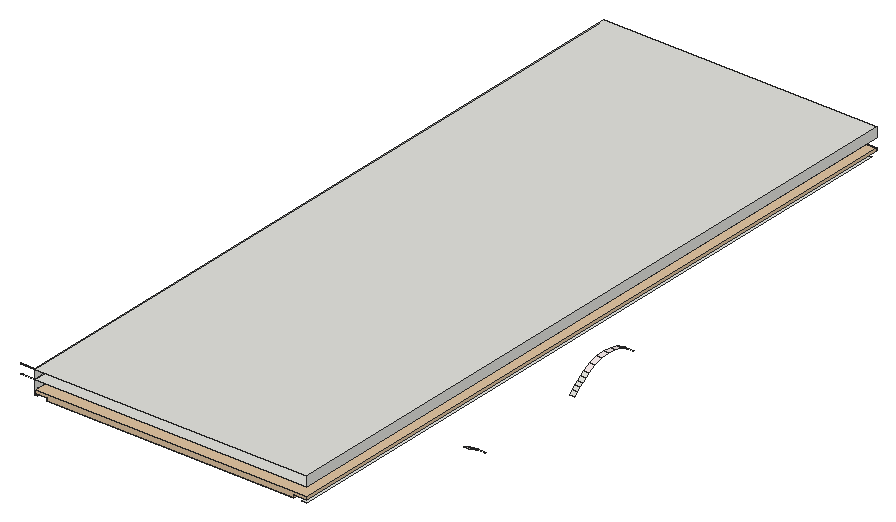
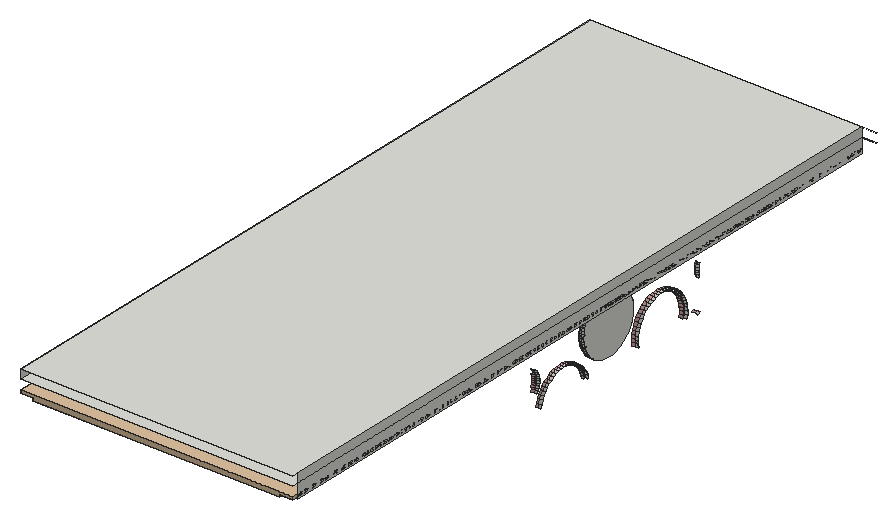
# SketchUp Ruby script. Lengths in inches.
U = 1.inch
M = Sketchup.active_model
def pt(a) = Geom::Point3d.new(a.map { |v| v * U })
def face(e, loops, mat)
  f = e.add_face(loops[0].map { |a| pt(a) })
  loops[1..].each { |l| e.add_face(l.map { |a| pt(a) }).erase! }
  f.material = f.back_material = mat if mat
  f
end
# faces: each face lists its corners as indices into pts; further lists are holes
def faces(e, pts, list, mat = nil) = list.each { |f| face(e, (f[0].is_a?(Array) ? f : [f]).map { |l| l.map { |i| pts[i] } }, mat) }
# xy, xz, yz: faces in a plane at the given z, y or x. An outline is a flat list of corners, or four numbers for a rectangle; further outlines are holes
def ring(l) = l.size == 4 ? [[l[0], l[1]], [l[2], l[1]], [l[2], l[3]], [l[0], l[3]]] : l.each_slice(2).to_a
def flat(e, list, mat, &to3) = list.each { |f| face(e, (f[0].is_a?(Array) ? f : [f]).map { |l| ring(l).map { |u, v| to3.(u, v) } }, mat) }
def xy(e, z, list, mat = nil) = flat(e, list, mat) { |x, y| [x, y, z] }
def xz(e, y, list, mat = nil) = flat(e, list, mat) { |x, z| [x, y, z] }
def yz(e, x, list, mat = nil) = flat(e, list, mat) { |y, z| [x, y, z] }
def lines(e, pts, list) = list.each { |a, b| e.add_line(pt(pts[a]), pt(pts[b])) }
# prism: a flat outline (further loops are holes) pulled along v
def prism(e, loops, v, mat = nil)
  f = face(e, loops, mat); d = Geom::Vector3d.new(v.map { |x| x * U })
  f.pushpull(f.normal.samedirection?(d) ? d.length : -d.length)
end
def box(e, o, s, mat = nil) = prism(e, [[o, [o[0] + s[0], o[1], o[2]], [o[0] + s[0], o[1] + s[1], o[2]], [o[0], o[1] + s[1], o[2]]]], [0, 0, s[2]], mat)
def at(x, y, z, deg = 0) = Geom::Transformation.translation(pt([x, y, z])) * Geom::Transformation.rotation(ORIGIN, Z_AXIS, deg.degrees)
def axes(o, x, y, z) = Geom::Transformation.new([*x, 0, *y, 0, *z, 0, *pt(o).to_a, 1])
def part(name) = M.definitions.add(name)
# library, detail: a bought-in or finely detailed component or shape, given as its bounding box
def library(name, o, s) = part(name).tap { |d| box(d.entities, o, s) }
def detail(e, o, s) = box(e.add_group.entities, o, s)
def put(e, d, t, mat = nil) = e.add_instance(d, t).tap { |i| i.material = mat if mat }
def group(e, t, mat = nil) = e.add_group.tap { |g| g.transformation = t; g.material = mat if mat }.entities
root = M.entities
M.materials.add("Generic").color = [224, 169, 169]
M.materials.add("Generic\#2").color = [246, 234, 234]
M.materials.add("Generic\#3").color = [224, 196, 161]
M.materials.add("[Mirror 01]").color = [185, 185, 185]
xy(root,120,[[180.9375,0,184.0625,453.375],[9,0.4375,10.6875,0.4375,10.6875,106.01,11.4375,106.01,11.4375,107.97,10.6875,107.97,10.6875,125.48,11.4375,125.48,11.4375,127.43,10.6875,127.43,10.6875,185.75,12.375,185.75,12.375,188.375,10.6875,188.375,10.6875,218.875,12.375,218.875,12.375,221.5,10.6875,221.5,10.6875,295.22,12.1875,295.22,12.1875,297.72,10.6875,297.72,10.6875,330.66,12.1875,330.66,12.1875,333.16,10.6875,333.16,10.6875,453.375,9,453.375]])
xy(root,129.25,[[0,0,0,0.4375,9,0.4375,9,457.3,184.0625,457.3,184.0625,0]])
xy(root,135.25,[[0,0,184.0625,0,184.0625,457.3,9,457.3,9,0.4375,0,0.4375]])
yz(root,9,[[203.625,92.14,205.19,92.2,206.74,92.38,208.27,92.69,209.77,93.12,211.23,93.67,212.64,94.33,214,95.1,215.29,95.97,216.51,96.95,217.65,98.02,218.7,99.17,219.66,100.41,220.51,101.71,221.26,103.08,221.89,104.51,222.42,105.98,222.82,107.49,223.1,109.02,223.26,110.58,223.3,112.14,223.21,113.7,223,115.24,222.66,116.77,222.21,118.26,221.64,119.71,221.5,120,185.75,120,185.61,119.71,185.04,118.26,184.59,116.77,184.25,115.24,184.04,113.7,183.95,112.14,183.99,110.58,184.15,109.02,184.43,107.49,184.84,105.98,185.36,104.51,185.99,103.08,186.74,101.71,187.6,100.41,188.55,99.17,189.6,98.02,190.74,96.95,191.96,95.97,193.25,95.1,194.61,94.33,196.02,93.67,197.48,93.12,198.99,92.69,200.52,92.38,202.07,92.2],[0.4375,120,453.375,129.25],[0.4375,129.25,453.375,135.25]])
yz(root,10.6875,[[203.625,94.5,205,94.55,206.36,94.72,207.71,94.99,209.03,95.37,210.32,95.85,211.5625,96.43,212.76,97.1,213.89,97.875,214.97,98.73,215.97,99.67,216.89,100.6875,217.73,101.78,218.48,102.93,219.14,104.13,219.7,105.39,220.16,106.68,220.51,108.01,220.76,109.36,220.9,110.72,220.93,112.1,220.86,113.47,220.67,114.83,220.375,116.17,219.98,117.49,219.48,118.77,218.875,120,188.375,120,187.77,118.77,187.27,117.49,186.875,116.17,186.58,114.83,186.4,113.47,186.32,112.1,186.35,110.72,186.49,109.36,186.74,108.01,187.09,106.68,187.55,105.39,188.11,104.13,188.77,102.93,189.52,101.78,190.36,100.6875,191.28,99.67,192.29,98.73,193.36,97.875,194.5,97.1,195.69,96.43,196.93,95.85,198.22,95.37,199.54,94.99,200.89,94.72,202.25,94.55]],"[Mirror 01]")
yz(root,12.375,[[203.625,92.14,205.19,92.2,206.74,92.38,208.27,92.69,209.77,93.12,211.23,93.67,212.64,94.33,214,95.1,215.29,95.97,216.51,96.95,217.65,98.02,218.7,99.17,219.66,100.41,220.51,101.71,221.26,103.08,221.89,104.51,222.42,105.98,222.82,107.49,223.1,109.02,223.26,110.58,223.3,112.14,223.21,113.7,223,115.24,222.66,116.77,222.21,118.26,221.64,119.71,221.5,120,218.875,120,219.48,118.77,219.98,117.49,220.375,116.17,220.67,114.83,220.86,113.47,220.93,112.1,220.9,110.72,220.76,109.36,220.51,108.01,220.16,106.68,219.7,105.39,219.14,104.13,218.48,102.93,217.73,101.78,216.89,100.6875,215.97,99.67,214.97,98.73,213.89,97.875,212.76,97.1,211.5625,96.43,210.32,95.85,209.03,95.37,207.71,94.99,206.36,94.72,205,94.55,203.625,94.5,202.25,94.55,200.89,94.72,199.54,94.99,198.22,95.37,196.93,95.85,195.69,96.43,194.5,97.1,193.36,97.875,192.29,98.73,191.28,99.67,190.36,100.6875,189.52,101.78,188.77,102.93,188.11,104.13,187.55,105.39,187.09,106.68,186.74,108.01,186.49,109.36,186.35,110.72,186.32,112.1,186.4,113.47,186.58,114.83,186.875,116.17,187.27,117.49,187.77,118.77,188.375,120,185.75,120,185.61,119.71,185.04,118.26,184.59,116.77,184.25,115.24,184.04,113.7,183.95,112.14,183.99,110.58,184.15,109.02,184.43,107.49,184.84,105.98,185.36,104.51,185.99,103.08,186.74,101.71,187.6,100.41,188.55,99.17,189.6,98.02,190.74,96.95,191.96,95.97,193.25,95.1,194.61,94.33,196.02,93.67,197.48,93.12,198.99,92.69,200.52,92.38,202.07,92.2]],"Generic")
yz(root,184.0625,[[0,129.25,457.3,135.25]])
p = [[10.6875,131.75,85.21],[10.6875,130.28,85.99],[9,130.28,85.99],[9,131.75,85.21],[12.9375,130.28,85.99],[12.9375,131.75,85.21],
  [184.0625,143.35,85.58],[184.0625,140.15,87.99],[180.9375,140.15,87.99],[180.9375,143.35,85.58],[10.6875,256.25,88.14],[10.6875,256.74,86.13],
  [12.1875,256.74,86.13],[12.1875,256.25,88.14],[184.0625,217.14,88.18],[184.0625,214.93,86.28],[180.9375,214.93,86.28],[180.9375,217.14,88.18],
  [10.6875,257.93,86.34],[10.6875,257.41,88.49],[9,257.41,88.49],[9,257.93,86.34],[12.1875,257.41,88.49],[12.1875,257.93,86.34],
  [10.6875,140.51,88.69],[10.6875,140.86,86.45],[9,140.86,86.45],[9,140.51,88.69],[13,140.86,86.45],[13,140.51,88.69],
  [10.6875,142.23,86.75],[10.6875,141.9,88.83],[13,141.9,88.83],[13,142.23,86.75],[10.6875,179.76,86.9],[10.6875,180.06,89.14],
  [9,180.06,89.14],[9,179.76,86.9],[13,180.06,89.14],[13,179.76,86.9],[10.6875,221.22,86.86],[10.6875,221.78,88.85],
  [12.1875,221.78,88.85],[12.1875,221.22,86.86],[10.6875,220.64,89.25],[10.6875,220.03,87.125],[9,220.03,87.125],[9,220.64,89.25],
  [12.1875,220.03,87.125],[12.1875,220.64,89.25],[10.6875,178.66,89.25],[10.6875,178.39,87.16],[13,178.39,87.16],[13,178.66,89.25],
  [184.0625,136.83,90.22],[180.9375,136.83,90.22],[10.6875,255.54,90.08],[12.1875,255.54,90.08],[184.0625,219.41,90.01],[180.9375,219.41,90.01],
  [10.6875,256.66,90.5625],[9,256.66,90.5625],[12.1875,256.66,90.5625],[10.6875,140.42,90.96],[9,140.42,90.96],[13,140.42,90.96],
  [10.6875,141.82,90.93],[13,141.82,90.93],[10.6875,222.57,90.76],[12.1875,222.57,90.76],[10.6875,180.1,91.41],[9,180.1,91.41],
  [13,180.1,91.41],[10.6875,178.7,91.35],[13,178.7,91.35],[10.6875,221.48,91.29],[9,221.48,91.29],[12.1875,221.48,91.29],
  [184.0625,221.73,91.77],[180.9375,221.73,91.77],[10.6875,254.61,91.93],[12.1875,254.61,91.93],[184.0625,133.39,92.26],[180.9375,133.39,92.26],
  [10.6875,255.67,92.54],[9,255.67,92.54],[12.1875,255.67,92.54],[10.6875,223.58,92.57],[12.1875,223.58,92.57],[10.6875,141.98,93.03],
  [13,141.98,93.03],[10.6875,140.59,93.22],[9,140.59,93.22],[13,140.59,93.22],[10.6875,222.55,93.22],[9,222.55,93.22],
  [12.1875,222.55,93.22],[10.6875,178.49,93.45],[13,178.49,93.45],[10.6875,179.88,93.66],[9,179.88,93.66],[13,179.88,93.66],
  [184.0625,224.11,93.46],[180.9375,224.11,93.46],[10.6875,253.48,93.66],[12.1875,253.48,93.66],[184.0625,262.21,91.98],[184.0625,257.84,95.3125],
  [180.9375,257.84,95.3125],[180.9375,262.21,91.98],[10.6875,202.07,92.2],[10.6875,203.625,92.14],[9,203.625,92.14],[9,202.07,92.2],
  [12.375,203.625,92.14],[12.375,202.07,92.2],[10.6875,205.19,92.2],[9,205.19,92.2],[12.375,205.19,92.2],[10.6875,200.52,92.38],
  [9,200.52,92.38],[12.375,200.52,92.38],[10.6875,206.74,92.38],[9,206.74,92.38],[12.375,206.74,92.38],[184.0625,129.85,94.12],
  [180.9375,129.85,94.12],[10.6875,198.99,92.69],[9,198.99,92.69],[12.375,198.99,92.69],[10.6875,208.27,92.69],[9,208.27,92.69],
  [12.375,208.27,92.69],[10.6875,254.46,94.39],[9,254.46,94.39],[12.1875,254.46,94.39],[10.6875,224.78,94.26],[12.1875,224.78,94.26],
  [10.6875,197.48,93.12],[9,197.48,93.12],[12.375,197.48,93.12],[10.6875,209.77,93.12],[9,209.77,93.12],[12.375,209.77,93.12],
  [10.6875,142.37,95.1],[13,142.37,95.1],[10.6875,196.02,93.67],[9,196.02,93.67],[12.375,196.02,93.67],[10.6875,211.23,93.67],
  [9,211.23,93.67],[12.375,211.23,93.67],[10.6875,141.01,95.44],[9,141.01,95.44],[13,141.01,95.44],[10.6875,223.83,95.02],
  [9,223.83,95.02],[12.1875,223.83,95.02],[10.6875,178.05,95.51],[13,178.05,95.51],[184.0625,226.54,95.08],[180.9375,226.54,95.08],
  [10.6875,179.4,95.88],[9,179.4,95.88],[13,179.4,95.88],[10.6875,194.61,94.33],[9,194.61,94.33],[12.375,194.61,94.33],
  [10.6875,212.64,94.33],[9,212.64,94.33],[12.375,212.64,94.33],[10.6875,252.16,95.26],[12.1875,252.16,95.26],[10.6875,193.25,95.1],
  [9,193.25,95.1],[12.375,193.25,95.1],[10.6875,214,95.1],[9,214,95.1],[12.375,214,95.1],[10.6875,226.17,95.79],
  [12.1875,226.17,95.79],[10.6875,253.05,96.08],[9,253.05,96.08],[12.1875,253.05,96.08],[10.6875,203.625,94.5],[10.6875,202.25,94.55],
  [12.375,202.25,94.55],[12.375,203.625,94.5],[10.6875,205,94.55],[12.375,205,94.55],[10.6875,200.89,94.72],[12.375,200.89,94.72],
  [10.6875,206.36,94.72],[12.375,206.36,94.72],[10.6875,199.54,94.99],[12.375,199.54,94.99],[10.6875,207.71,94.99],[12.375,207.71,94.99],
  [10.6875,198.22,95.37],[12.375,198.22,95.37],[10.6875,209.03,95.37],[12.375,209.03,95.37],[10.6875,225.3125,96.66],[9,225.3125,96.66],
  [12.1875,225.3125,96.66],[10.6875,143,97.11],[13,143,97.11],[10.6875,191.96,95.97],[9,191.96,95.97],[12.375,191.96,95.97],
  [10.6875,215.29,95.97],[9,215.29,95.97],[12.375,215.29,95.97],[184.0625,231.42,97.61],[180.9375,231.42,97.61],[10.6875,250.66,96.6875],
  [12.1875,250.66,96.6875],[184.0625,252.92,97.77],[180.9375,252.92,97.77],[10.6875,141.6875,97.61],[9,141.6875,97.61],[13,141.6875,97.61],
  [10.6875,196.93,95.85],[12.375,196.93,95.85],[10.6875,210.32,95.85],[12.375,210.32,95.85],[10.6875,177.38,97.5],[13,177.38,97.5],
  [10.6875,195.69,96.43],[12.375,195.69,96.43],[10.6875,211.5625,96.43],[12.375,211.5625,96.43],[10.6875,227.72,97.16],[12.1875,227.72,97.16],
  [10.6875,178.68,98.03],[9,178.68,98.03],[13,178.68,98.03],[10.6875,190.74,96.95],[9,190.74,96.95],[12.375,190.74,96.95],
  [10.6875,216.51,96.95],[9,216.51,96.95],[12.375,216.51,96.95],[10.6875,251.45,97.61],[9,251.45,97.61],[12.1875,251.45,97.61],
  [10.6875,260.36,97.44],[10.6875,261.03,96.23],[9,261.03,96.23],[9,260.36,97.44],[12.9375,261.03,96.23],[12.9375,260.36,97.44],
  [10.6875,194.5,97.1],[12.375,194.5,97.1],[10.6875,212.76,97.1],[12.375,212.76,97.1],[10.6875,226.97,98.12],[9,226.97,98.12],
  [12.1875,226.97,98.12],[10.6875,249.01,97.9375],[12.1875,249.01,97.9375],[10.6875,189.6,98.02],[9,189.6,98.02],[12.375,189.6,98.02],
  [10.6875,217.65,98.02],[9,217.65,98.02],[12.375,217.65,98.02],[10.6875,143.85,99.04],[13,143.85,99.04],[10.6875,193.36,97.875],
  [12.375,193.36,97.875],[10.6875,213.89,97.875],[12.375,213.89,97.875],[10.6875,229.42,98.34],[12.1875,229.42,98.34],[10.6875,259.83,98.73],
  [9,259.83,98.73],[12.9375,259.83,98.73],[10.6875,176.48,99.41],[13,176.48,99.41],[10.6875,142.61,99.68],[9,142.61,99.68],
  [13,142.61,99.68],[184.0625,236.6875,99.18],[180.9375,236.6875,99.18],[10.6875,249.69,98.95],[9,249.69,98.95],[12.1875,249.69,98.95],
  [184.0625,247.63,99.26],[180.9375,247.63,99.26],[10.6875,192.29,98.73],[12.375,192.29,98.73],[10.6875,214.97,98.73],[12.375,214.97,98.73],
  [10.6875,247.23,98.99],[12.1875,247.23,98.99],[10.6875,177.71,100.08],[9,177.71,100.08],[13,177.71,100.08],[10.6875,188.55,99.17],
  [9,188.55,99.17],[12.375,188.55,99.17],[10.6875,218.7,99.17],[9,218.7,99.17],[12.375,218.7,99.17],[10.6875,228.78,99.38],
  [9,228.78,99.38],[12.1875,228.78,99.38],[10.6875,231.24,99.32],[12.1875,231.24,99.32],[10.6875,191.28,99.67],[12.375,191.28,99.67],
  [10.6875,215.97,99.67],[12.375,215.97,99.67],[10.6875,259.45,100.07],[9,259.45,100.07],[12.9375,259.45,100.07],[10.6875,247.79,100.07],
  [9,247.79,100.07],[12.1875,247.79,100.07],[10.6875,144.92,100.86],[13,144.92,100.86],[10.6875,245.34,99.84],[12.1875,245.34,99.84],
  [10.6875,187.6,100.41],[9,187.6,100.41],[12.375,187.6,100.41],[10.6875,219.66,100.41],[9,219.66,100.41],[12.375,219.66,100.41],
  [184.0625,242.16,99.73],[180.9375,242.16,99.73],[10.6875,261.07,99.16],[10.6875,260.73,100.35],[12.9375,260.73,100.35],[12.9375,261.07,99.16],
  [10.6875,233.16,100.09],[12.1875,233.16,100.09],[10.6875,175.375,101.2],[13,175.375,101.2],[10.6875,230.73,100.42],[9,230.73,100.42],
  [12.1875,230.73,100.42],[10.6875,143.75,101.63],[9,143.75,101.63],[13,143.75,101.63],[10.6875,190.36,100.6875],[12.375,190.36,100.6875],
  [10.6875,216.89,100.6875],[12.375,216.89,100.6875],[10.6875,243.37,100.46],[12.1875,243.37,100.46],[10.6875,176.52,102.01],[9,176.52,102.01],
  [13,176.52,102.01],[10.6875,235.16,100.63],[12.1875,235.16,100.63],[10.6875,245.78,100.97],[9,245.78,100.97],[12.1875,245.78,100.97],
  [10.6875,259.23,101.44],[9,259.23,101.44],[12.9375,259.23,101.44],[10.6875,186.74,101.71],[9,186.74,101.71],[12.375,186.74,101.71],
  [10.6875,220.51,101.71],[9,220.51,101.71],[12.375,220.51,101.71],[10.6875,232.78,101.24],[9,232.78,101.24],[12.1875,232.78,101.24],
  [10.6875,260.53,101.58],[12.9375,260.53,101.58],[10.6875,241.34,100.86],[12.1875,241.34,100.86],[10.6875,237.21,100.94],[12.1875,237.21,100.94],
  [10.6875,189.52,101.78],[12.375,189.52,101.78],[10.6875,217.73,101.78],[12.375,217.73,101.78],[10.6875,146.1875,102.54],[13,146.1875,102.54],
  [10.6875,239.28,101.02],[12.1875,239.28,101.02],[10.6875,243.67,101.64],[9,243.67,101.64],[12.1875,243.67,101.64],[10.6875,174.07,102.85],
  [13,174.07,102.85],[10.6875,234.91,101.82],[9,234.91,101.82],[12.1875,234.91,101.82],[10.6875,259.17,102.83],[9,259.17,102.83],
  [12.9375,259.17,102.83],[10.6875,145.12,103.44],[9,145.12,103.44],[13,145.12,103.44],[10.6875,241.5,102.06],[9,241.5,102.06],
  [12.1875,241.5,102.06],[10.6875,260.47,102.82],[12.9375,260.47,102.82],[10.6875,185.99,103.08],[9,185.99,103.08],[12.375,185.99,103.08],
  [10.6875,221.26,103.08],[9,221.26,103.08],[12.375,221.26,103.08],[10.6875,188.77,102.93],[12.375,188.77,102.93],[10.6875,218.48,102.93],
  [12.375,218.48,102.93],[10.6875,237.09,102.15],[9,237.09,102.15],[12.1875,237.09,102.15],[10.6875,175.12,103.78],[9,175.12,103.78],
  [13,175.12,103.78],[10.6875,239.3,102.23],[9,239.3,102.23],[12.1875,239.3,102.23],[10.6875,147.64,104.07],[13,147.64,104.07],
  [10.6875,259.26,104.22],[9,259.26,104.22],[12.9375,259.26,104.22],[10.6875,260.56,104.06],[12.9375,260.56,104.06],[10.6875,172.58,104.35],
  [13,172.58,104.35],[10.6875,188.11,104.13],[12.375,188.11,104.13],[10.6875,219.14,104.13],[12.375,219.14,104.13],[10.6875,185.36,104.51],
  [9,185.36,104.51],[12.375,185.36,104.51],[10.6875,221.89,104.51],[9,221.89,104.51],[12.375,221.89,104.51],[10.6875,146.68,105.09],
  [9,146.68,105.09],[13,146.68,105.09],[10.6875,173.52,105.39],[9,173.52,105.39],[13,173.52,105.39],[10.6875,149.25,105.42],
  [13,149.25,105.42],[10.6875,187.55,105.39],[12.375,187.55,105.39],[10.6875,219.7,105.39],[12.375,219.7,105.39],[10.6875,260.78,105.28],
  [12.9375,260.78,105.28],[10.6875,259.51,105.59],[9,259.51,105.59],[12.9375,259.51,105.59],[10.6875,170.9375,105.66],[13,170.9375,105.66],
  [10.6875,184.84,105.98],[9,184.84,105.98],[12.375,184.84,105.98],[10.6875,222.42,105.98],[9,222.42,105.98],[12.375,222.42,105.98],
  [10.6875,148.42,106.54],[9,148.42,106.54],[13,148.42,106.54],[10.6875,261.14,106.47],[12.9375,261.14,106.47],[10.6875,151.01,106.58],
  [13,151.01,106.58],[10.6875,171.75,106.81],[9,171.75,106.81],[13,171.75,106.81],[10.6875,187.09,106.68],[12.375,187.09,106.68],
  [10.6875,220.16,106.68],[12.375,220.16,106.68],[10.6875,259.92,106.92],[9,259.92,106.92],[12.9375,259.92,106.92],[10.6875,169.15,106.78],
  [13,169.15,106.78],[10.6875,184.43,107.49],[9,184.43,107.49],[12.375,184.43,107.49],[10.6875,222.82,107.49],[9,222.82,107.49],
  [12.375,222.82,107.49],[10.6875,130.9,106.11],[10.6875,131.2,107.5],[9,131.2,107.5],[9,130.9,106.11],[11.4375,131.2,107.5],
  [11.4375,130.9,106.11],[10.6875,150.31,107.79],[9,150.31,107.79],[13,150.31,107.79],[10.6875,152.89,107.53],[13,152.89,107.53],
  [10.6875,186.74,108.01],[12.375,186.74,108.01],[10.6875,220.51,108.01],[12.375,220.51,108.01],[10.6875,167.25,107.69],[13,167.25,107.69],
  [10.6875,169.83,108.01],[9,169.83,108.01],[13,169.83,108.01],[10.6875,260.47,108.19],[9,260.47,108.19],[12.9375,260.47,108.19],
  [10.6875,131.375,108.91],[9,131.375,108.91],[11.4375,131.375,108.91],[10.6875,154.87,108.26],[13,154.87,108.26],[10.6875,184.15,109.02],
  [9,184.15,109.02],[12.375,184.15,109.02],[10.6875,223.1,109.02],[9,223.1,109.02],[12.375,223.1,109.02],[10.6875,165.26,108.375],
  [13,165.26,108.375],[10.6875,152.33,108.8125],[9,152.33,108.8125],[13,152.33,108.8125],[10.6875,167.78,108.99],[9,167.78,108.99],
  [13,167.78,108.99],[10.6875,186.49,109.36],[12.375,186.49,109.36],[10.6875,220.76,109.36],[12.375,220.76,109.36],[10.6875,261.17,109.4],
  [9,261.17,109.4],[12.9375,261.17,109.4],[10.6875,156.91,108.76],[13,156.91,108.76],[10.6875,163.2,108.83],[13,163.2,108.83],
  [10.6875,154.46,109.6],[9,154.46,109.6],[13,154.46,109.6],[10.6875,159,109.02],[13,159,109.02],[10.6875,161.11,109.05],
  [13,161.11,109.05],[10.6875,131.41,110.32],[9,131.41,110.32],[11.4375,131.41,110.32],[10.6875,165.64,109.72],[9,165.64,109.72],
  [13,165.64,109.72],[10.6875,183.99,110.58],[9,183.99,110.58],[12.375,183.99,110.58],[10.6875,223.26,110.58],[9,223.26,110.58],
  [12.375,223.26,110.58],[10.6875,186.35,110.72],[12.375,186.35,110.72],[10.6875,220.9,110.72],[12.375,220.9,110.72],[10.6875,156.66,110.14],
  [9,156.66,110.14],[13,156.66,110.14],[10.6875,163.43,110.21],[9,163.43,110.21],[13,163.43,110.21],[10.6875,158.91,110.42],
  [9,158.91,110.42],[13,158.91,110.42],[10.6875,161.17,110.44],[9,161.17,110.44],[13,161.17,110.44],[10.6875,131.31,111.74],
  [9,131.31,111.74],[11.4375,131.31,111.74],[10.6875,183.95,112.14],[9,183.95,112.14],[12.375,183.95,112.14],[10.6875,223.3,112.14],
  [9,223.3,112.14],[12.375,223.3,112.14],[10.6875,186.32,112.1],[12.375,186.32,112.1],[10.6875,220.93,112.1],[12.375,220.93,112.1],
  [10.6875,131.07,113.14],[9,131.07,113.14],[11.4375,131.07,113.14],[10.6875,184.04,113.7],[9,184.04,113.7],[12.375,184.04,113.7],
  [10.6875,186.4,113.47],[12.375,186.4,113.47],[10.6875,220.86,113.47],[12.375,220.86,113.47],[10.6875,223.21,113.7],[9,223.21,113.7],
  [12.375,223.21,113.7],[10.6875,130.69,114.51],[9,130.69,114.51],[11.4375,130.69,114.51],[10.6875,186.58,114.83],[12.375,186.58,114.83],
  [10.6875,220.67,114.83],[12.375,220.67,114.83],[10.6875,184.25,115.24],[9,184.25,115.24],[12.375,184.25,115.24],[10.6875,223,115.24],
  [9,223,115.24],[12.375,223,115.24],[10.6875,186.875,116.17],[12.375,186.875,116.17],[10.6875,220.375,116.17],[12.375,220.375,116.17],
  [10.6875,184.59,116.77],[9,184.59,116.77],[12.375,184.59,116.77],[10.6875,222.66,116.77],[9,222.66,116.77],[12.375,222.66,116.77],
  [10.6875,187.27,117.49],[12.375,187.27,117.49],[10.6875,219.98,117.49],[12.375,219.98,117.49],[10.6875,185.04,118.26],[9,185.04,118.26],
  [12.375,185.04,118.26],[10.6875,222.21,118.26],[9,222.21,118.26],[12.375,222.21,118.26],[10.6875,187.77,118.77],[12.375,187.77,118.77],
  [10.6875,219.48,118.77],[12.375,219.48,118.77],[10.6875,185.61,119.71],[9,185.61,119.71],[12.375,185.61,119.71],[10.6875,221.64,119.71],
  [9,221.64,119.71],[12.375,221.64,119.71],[10.6875,188.375,120],[12.375,188.375,120],[10.6875,218.875,120],[12.375,218.875,120],
  [10.6875,185.75,120],[12.375,185.75,120],[10.6875,221.5,120],[12.375,221.5,120]]
faces(root,p,[[0,1,2,3],[14,15,16,17],[18,19,20,21],[24,25,26,27],[34,35,36,37],[44,45,46,47],[58,14,17,59],[19,60,61,20],
  [63,24,27,64],[35,70,71,36],[75,44,47,76],[78,58,59,79],[60,84,85,61],[91,63,64,92],[94,75,76,95],[70,99,100,71],
  [102,78,79,103],[110,111,112,113],[111,116,117,112],[119,110,113,120],[116,122,123,117],[127,119,120,128],[122,130,131,123],[84,133,134,85],
  [138,127,128,139],[130,141,142,131],[146,138,139,147],[141,149,150,142],[152,91,92,153],[155,94,95,156],[160,102,103,161],[99,162,163,100],
  [165,146,147,166],[149,168,169,150],[173,165,166,174],[168,176,177,169],[133,181,182,134],[202,155,156,203],[207,173,174,208],[176,210,211,177],
  [219,152,153,220],[162,234,235,163],[237,207,208,238],[210,240,241,211],[181,243,244,182],[246,247,248,249],[256,202,203,257],[261,237,238,262],
  [240,264,265,241],[275,246,249,276],[280,219,220,281],[243,285,286,244],[234,296,297,235],[299,261,262,300],[264,302,303,265],[305,256,257,306],
  [314,275,276,315],[285,317,318,286],[324,299,300,325],[302,327,328,303],[340,305,306,341],[343,280,281,344],[296,352,353,297],[317,357,358,318],
  [360,314,315,361],[363,324,325,364],[327,366,367,328],[369,340,341,370],[357,386,387,358],[391,369,370,392],[394,360,361,395],[397,343,344,398],
  [386,400,401,387],[405,363,364,406],[366,408,409,367],[415,391,392,416],[352,418,419,353],[400,421,422,401],[421,415,416,422],[426,394,395,427],
  [437,405,406,438],[408,440,441,409],[443,397,398,444],[418,446,447,419],[457,426,427,458],[462,437,438,463],[440,465,466,441],[468,443,444,469],
  [446,475,476,447],[482,457,458,483],[487,462,463,488],[465,490,491,466],[493,494,495,496],[499,468,469,500],[475,510,511,476],[513,482,483,514],
  [494,516,517,495],[521,487,488,522],[490,524,525,491],[529,499,500,530],[510,532,533,511],[539,513,514,540],[546,529,530,547],[516,553,554,517],
  [532,556,557,533],[559,521,522,560],[524,562,563,525],[569,546,547,570],[556,572,573,557],[575,569,570,576],[572,578,579,573],[553,581,582,554],
  [578,575,576,579],[584,559,560,585],[562,587,588,563],[581,594,595,582],[597,584,585,598],[587,604,605,588],[594,607,608,595],[614,597,598,615],
  [604,617,618,605],[624,614,615,625],[617,627,628,618],[634,624,625,635],[627,637,638,628],[644,634,635,645],[637,647,648,638]])
faces(root,p,[[0,1,4,5],[10,11,12,13],[18,19,22,23],[24,25,28,29],[30,31,32,33],[34,35,38,39],[40,41,42,43],[44,45,48,49],
  [50,51,52,53],[56,10,13,57],[19,60,62,22],[63,24,29,65],[31,66,67,32],[41,68,69,42],[35,70,72,38],[73,50,53,74],
  [75,44,49,77],[80,56,57,81],[60,84,86,62],[68,87,88,69],[66,89,90,67],[91,63,65,93],[94,75,77,96],[97,73,74,98],
  [70,99,101,72],[104,80,81,105],[110,111,114,115],[111,116,118,114],[119,110,115,121],[116,122,124,118],[127,119,121,129],[122,130,132,124],
  [84,133,135,86],[87,136,137,88],[138,127,129,140],[130,141,143,132],[89,144,145,90],[146,138,140,148],[141,149,151,143],[152,91,93,154],
  [155,94,96,157],[158,97,98,159],[99,162,164,101],[165,146,148,167],[149,168,170,151],[171,104,105,172],[173,165,167,175],[168,176,178,170],
  [136,179,180,137],[133,181,183,135],[184,185,186,187],[188,184,187,189],[185,190,191,186],[192,188,189,193],[190,194,195,191],[196,192,193,197],
  [194,198,199,195],[200,196,197,201],[202,155,157,204],[144,205,206,145],[207,173,175,209],[176,210,212,178],[215,171,172,216],[219,152,154,221],
  [198,222,223,199],[224,200,201,225],[226,158,159,227],[222,228,229,223],[230,224,225,231],[179,232,233,180],[162,234,236,164],[237,207,209,239],
  [210,240,242,212],[181,243,245,183],[246,247,250,251],[228,252,253,229],[254,230,231,255],[256,202,204,258],[259,215,216,260],[261,237,239,263],
  [240,264,266,242],[205,267,268,206],[252,269,270,253],[271,254,255,272],[232,273,274,233],[275,246,251,277],[278,226,227,279],[280,219,221,282],
  [243,285,287,245],[269,290,291,270],[292,271,272,293],[294,259,260,295],[234,296,298,236],[299,261,263,301],[264,302,304,266],[305,256,258,307],
  [273,308,309,274],[290,310,311,291],[312,292,293,313],[314,275,277,316],[285,317,319,287],[267,320,321,268],[322,294,295,323],[324,299,301,326],
  [302,327,329,304],[332,333,334,335],[308,336,337,309],[338,278,279,339],[340,305,307,342],[343,280,282,345],[310,346,347,311],[348,312,313,349],
  [350,322,323,351],[296,352,354,298],[336,355,356,337],[317,357,359,319],[360,314,316,362],[363,324,326,365],[327,366,368,329],[369,340,342,371],
  [333,372,373,334],[374,350,351,375],[355,376,377,356],[346,378,379,347],[380,348,349,381],[320,382,383,321],[376,384,385,377],[384,374,375,385],
  [357,386,388,359],[389,338,339,390],[391,369,371,393],[394,360,362,396],[397,343,345,399],[386,400,402,388],[372,403,404,373],[405,363,365,407],
  [366,408,410,368],[378,411,412,379],[413,380,381,414],[415,391,393,417],[352,418,420,354],[400,421,423,402],[421,415,417,423],[382,424,425,383],
  [426,394,396,428],[403,429,430,404],[431,389,390,432],[411,433,434,412],[435,413,414,436],[437,405,407,439],[408,440,442,410],[443,397,399,445],
  [418,446,448,420],[424,449,450,425],[433,451,452,434],[453,435,436,454],[429,455,456,430],[457,426,428,459],[460,431,432,461],[462,437,439,464],
  [440,465,467,442],[468,443,445,470],[455,471,472,456],[449,473,474,450],[446,475,477,448],[451,478,479,452],[480,453,454,481],[482,457,459,484],
  [485,460,461,486],[487,462,464,489],[465,490,492,467],[493,494,497,498],[499,468,470,501],[473,502,503,474],[478,504,505,479],[506,480,481,507],
  [508,485,486,509],[475,510,512,477],[513,482,484,515],[494,516,518,497],[502,519,520,503],[521,487,489,523],[490,524,526,492],[527,508,509,528],
  [529,499,501,531],[510,532,534,512],[504,535,536,505],[537,506,507,538],[539,513,515,541],[519,542,543,520],[544,527,528,545],[546,529,531,548],
  [542,549,550,543],[551,544,545,552],[516,553,555,518],[549,551,552,550],[532,556,558,534],[559,521,523,561],[524,562,564,526],[535,565,566,536],
  [567,537,538,568],[569,546,548,571],[556,572,574,558],[575,569,571,577],[572,578,580,574],[553,581,583,555],[578,575,577,580],[584,559,561,586],
  [562,587,589,564],[565,590,591,566],[592,567,568,593],[581,594,596,583],[597,584,586,599],[590,600,601,591],[602,592,593,603],[587,604,606,589],
  [594,607,609,596],[600,610,611,601],[612,602,603,613],[614,597,599,616],[604,617,619,606],[610,620,621,611],[622,612,613,623],[624,614,616,626],
  [617,627,629,619],[620,630,631,621],[632,622,623,633],[634,624,626,636],[627,637,639,629],[630,640,641,631],[642,632,633,643],[644,634,636,646],
  [637,647,649,639],[640,650,651,641],[652,642,643,653],[654,644,646,655],[647,656,657,649]],"Generic")
faces(root,p,[[6,7,8,9],[7,54,55,8],[54,82,83,55],[106,107,108,109],[82,125,126,83],[213,160,161,214],[107,217,218,108],[283,213,214,284],
  [217,288,289,218],[330,283,284,331],[288,330,331,289]],"Generic\#2")
g1 = group(root,at(0,0,119.9375),"Generic\#3")
xy(g1,0,[[17.33,0,175.73,457.3]])
xy(g1,1.5625,[[9,0,17.33,457.3],[175.73,0,184.0625,457.3]])
xy(g1,3.3125,[[9,0,184.0625,457.3]])
xz(g1,0,[[17.33,0,175.73,0,175.73,1.5625,184.0625,1.5625,184.0625,3.3125,9,3.3125,9,1.5625,17.33,1.5625]])
xz(g1,457.3,[[17.33,0,17.33,1.5625,9,1.5625,9,3.3125,184.0625,3.3125,184.0625,1.5625,175.73,1.5625,175.73,0]])
yz(g1,9,[[0,1.5625,453.375,3.3125],[453.375,1.5625,453.625,3.3125],[453.625,1.5625,457.3,3.3125]])
yz(g1,17.33,[[0,0,457.3,1.5625]])
yz(g1,175.73,[[0,0,457.3,1.5625]])
yz(g1,184.0625,[[0,1.5625,457.3,3.3125]])
p = [[0,0.4375,3.3125],[0,0,3.3125]]
lines(g1,p,[[0,1]])
